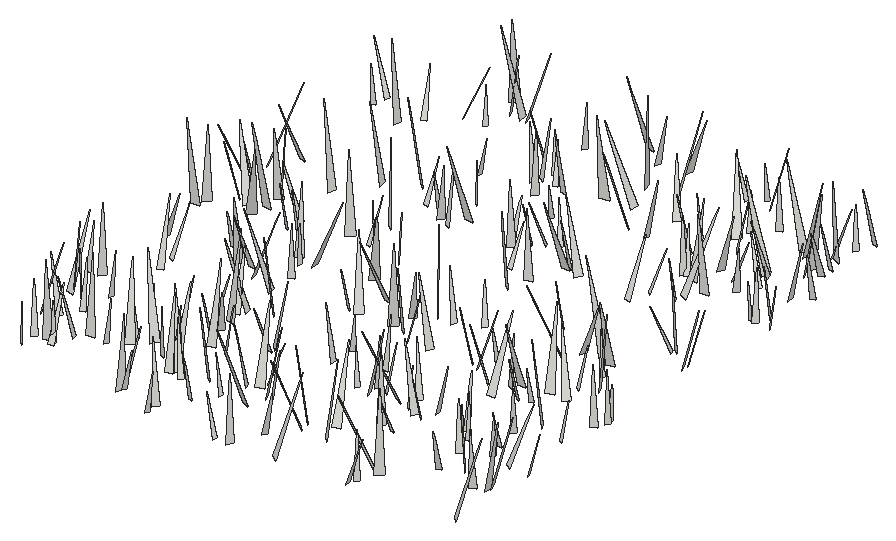
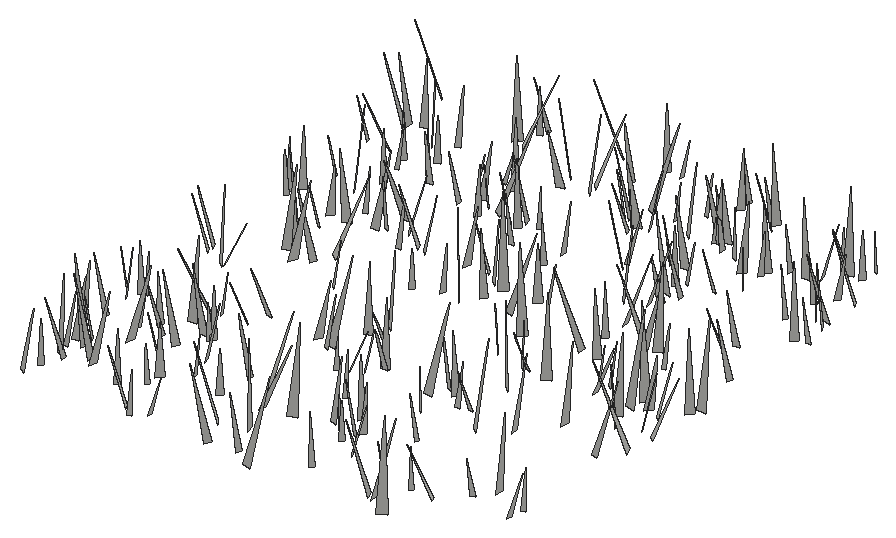
# SketchUp Ruby script. Lengths in inches.
U = 1.inch
M = Sketchup.active_model
def pt(a) = Geom::Point3d.new(a.map { |v| v * U })
def face(e, loops, mat)
  f = e.add_face(loops[0].map { |a| pt(a) })
  loops[1..].each { |l| e.add_face(l.map { |a| pt(a) }).erase! }
  f.material = f.back_material = mat if mat
  f
end
# faces: each face lists its corners as indices into pts; further lists are holes
def faces(e, pts, list, mat = nil) = list.each { |f| face(e, (f[0].is_a?(Array) ? f : [f]).map { |l| l.map { |i| pts[i] } }, mat) }
# xy, xz, yz: faces in a plane at the given z, y or x. An outline is a flat list of corners, or four numbers for a rectangle; further outlines are holes
def ring(l) = l.size == 4 ? [[l[0], l[1]], [l[2], l[1]], [l[2], l[3]], [l[0], l[3]]] : l.each_slice(2).to_a
def flat(e, list, mat, &to3) = list.each { |f| face(e, (f[0].is_a?(Array) ? f : [f]).map { |l| ring(l).map { |u, v| to3.(u, v) } }, mat) }
def xy(e, z, list, mat = nil) = flat(e, list, mat) { |x, y| [x, y, z] }
def xz(e, y, list, mat = nil) = flat(e, list, mat) { |x, z| [x, y, z] }
def yz(e, x, list, mat = nil) = flat(e, list, mat) { |y, z| [x, y, z] }
def lines(e, pts, list) = list.each { |a, b| e.add_line(pt(pts[a]), pt(pts[b])) }
# prism: a flat outline (further loops are holes) pulled along v
def prism(e, loops, v, mat = nil)
  f = face(e, loops, mat); d = Geom::Vector3d.new(v.map { |x| x * U })
  f.pushpull(f.normal.samedirection?(d) ? d.length : -d.length)
end
def box(e, o, s, mat = nil) = prism(e, [[o, [o[0] + s[0], o[1], o[2]], [o[0] + s[0], o[1] + s[1], o[2]], [o[0], o[1] + s[1], o[2]]]], [0, 0, s[2]], mat)
def at(x, y, z, deg = 0) = Geom::Transformation.translation(pt([x, y, z])) * Geom::Transformation.rotation(ORIGIN, Z_AXIS, deg.degrees)
def axes(o, x, y, z) = Geom::Transformation.new([*x, 0, *y, 0, *z, 0, *pt(o).to_a, 1])
def part(name) = M.definitions.add(name)
# library, detail: a bought-in or finely detailed component or shape, given as its bounding box
def library(name, o, s) = part(name).tap { |d| box(d.entities, o, s) }
def detail(e, o, s) = box(e.add_group.entities, o, s)
def put(e, d, t, mat = nil) = e.add_instance(d, t).tap { |i| i.material = mat if mat }
def group(e, t, mat = nil) = e.add_group.tap { |g| g.transformation = t; g.material = mat if mat }.entities
root = M.entities
c1 = part("fur_instance\#9")
p = [[0.8125,0,1.79],[0.67,-0.02,1.48],[0,-0.11,0],[0,0.11,0]]
faces(c1.entities,p,[[0,1,2,3]])
put(root,c1,axes([490.36,55.36,-21.66],[3.76138,-1.24538,0.93866],[-1.27843,-3.86595,-0.00634],[-0.89313,0.28885,3.96218]))
put(root,c1,axes([503.76,55.4,-21.66],[-3.79892,0.58903,0.61511],[0.5899,3.84804,-0.04166],[0.61427,-0.05255,3.84409]))
put(root,c1,axes([506.5,55.57,-21.66],[-5.0872,2.66073,2.45988],[2.85923,5.55214,-0.09239],[2.22604,-1.05084,5.74025]))
put(root,c1,axes([528.55,57.22,-21.66],[4.6292,0.17151,0.50537],[0.17521,-4.6565,-0.02456],[-0.5041,-0.0434,4.63231]))
put(root,c1,axes([482.875,58.1875,-21.66],[-5.61419,2.77509,3.47904],[3.15086,6.4338,-0.04739],[3.14276,-1.49299,6.26243]))
put(root,c1,axes([490.25,57.73,-21.66],[-4.38445,3.57185,1.79964],[3.76738,4.58485,0.07863],[1.34299,-1.20052,5.65467]))
put(root,c1,axes([514.83,56.21,-21.66],[4.48947,6.23838,0.89691],[6.27438,-4.52789,0.08708],[-0.59503,-0.67674,7.68539]))
put(root,c1,axes([483.18,58.77,-21.66],[3.78435,-1.32179,0.68035],[-1.35222,-3.83372,0.07338],[-0.61764,0.29457,4.00787]))
put(root,c1,axes([529.15,58.78,-21.66],[1.67153,-3.68103,1.97281],[-4.08391,-1.88531,-0.05752],[-0.87388,1.76964,4.04237]))
put(root,c1,axes([461.67,60.13,-21.66],[1.95949,2.80373,1.45551],[3.04239,-2.136,0.01872],[-0.85045,-1.18135,3.42055]))
put(root,c1,axes([548.44,58.8,-21.66],[5.3088,5.05785,1.00754],[5.10033,-5.36326,0.04959],[-0.76398,-0.65873,7.33231]))
put(root,c1,axes([482.64,59.66,-21.66],[3.62084,3.81527,1.03017],[3.87963,-3.69771,0.05854],[-0.75237,-0.70613,5.25959]))
put(root,c1,axes([508.8125,61.37,-21.66],[3.98619,-2.41358,0.43201],[-2.42835,-4.00018,0.05811],[-0.33929,0.27366,4.65958]))
put(root,c1,axes([528.84,63.33,-21.66],[-5.75391,-4.14909,0.07824],[-4.14913,5.75437,0.02082],[0.07564,0.02888,7.0938]))
put(root,c1,axes([493.09,62.62,-21.66],[-1.22069,-3.41408,1.05948],[-3.55821,1.26785,-0.01408],[0.34288,1.00256,3.62571]))
put(root,c1,axes([530.64,62.39,-21.66],[5.17413,-4.7343,3.23528],[-5.24163,-5.67192,0.08293],[-2.32507,2.25121,7.01272]))
put(root,c1,axes([464.33,63.53,-21.66],[2.05152,-6.96349,2.48946],[-7.36809,-2.14532,0.07104],[-0.63146,2.40909,7.25905]))
put(root,c1,axes([465.36,63.47,-21.66],[2.21811,-2.97156,1.30139],[-3.14682,-2.35396,-0.01147],[-0.78819,1.03561,3.7081]))
put(root,c1,axes([461.8,63.27,-21.66],[2.76185,-3.07557,2.49035],[-3.57907,-3.23702,-0.02845],[-1.68858,1.83068,4.13354]))
put(root,c1,axes([512.22,66.18,-21.66],[-4.64993,-4.92524,0.42817],[-4.93518,4.6591,-0.00251],[0.29211,0.31306,6.77347]))
put(root,c1,axes([465.56,62.57,-21.66],[-0.62554,4.99616,0.12365],[4.99768,0.62512,0.02455],[-0.009,-0.12574,5.03511]))
put(root,c1,axes([500.61,66.83,-21.66],[-3.23676,-6.95107,0.75182],[-6.9834,3.25434,0.02332],[0.33861,0.67166,7.66769]))
put(root,c1,axes([466.89,66.75,-21.66],[-4.90354,-1.85753,0.89414],[-1.8937,4.97041,-0.05944],[0.81474,0.37312,5.24324]))
put(root,c1,axes([517.3,66.01,-21.66],[-4.33935,-4.28478,3.74469],[-5.00881,5.11096,0.04388],[2.70071,2.59437,6.09815]))
put(root,c1,axes([496.04,66.59,-21.66],[-3.46887,0.5768,0.94943],[0.60796,3.5911,0.03958],[0.92978,-0.19616,3.51628]))
put(root,c1,axes([544.63,68.05,-21.66],[1.69924,-5.28596,1.58911],[-5.50046,-1.7602,0.02657],[-0.46001,1.5213,5.5523]))
put(root,c1,axes([511.7,68.27,-21.66],[-4.72321,-4.87597,2.05821],[-5.0831,4.94763,0.05633],[1.47426,1.43735,6.78828]))
put(root,c1,axes([536.71,69.47,-21.66],[2.00782,-4.43373,0.05819],[-4.43409,-2.00742,0.0429],[0.01508,0.0707,4.86698]))
put(root,c1,axes([487.84,66.88,-21.66],[-3.61656,3.24074,0.55892],[3.26072,3.64166,-0.01623],[0.42715,-0.36083,4.85609]))
put(root,c1,axes([471.99,68.38,-21.66],[-3.43259,1.11019,2.13702],[1.24058,4.00441,-0.08763],[2.06406,-0.56053,3.60659]))
put(root,c1,axes([485.18,67.19,-21.66],[-1.64071,6.20292,1.41522],[6.35653,1.66047,0.09149],[0.27128,-1.39198,6.41559]))
put(root,c1,axes([468.6,68.52,-21.66],[-0.16128,6.84934,2.86842],[7.42417,0.20732,-0.07764],[0.15166,-2.86546,6.8508]))
put(root,c1,axes([491.39,69.34,-21.66],[-4.35453,-4.53446,2.05004],[-4.74623,4.60317,0.10013],[1.49574,1.4055,6.28595]))
put(root,c1,axes([546.7,69.05,-21.66],[6.13024,0.22864,1.74835],[0.20896,-6.37456,0.10097],[-1.75081,0.03976,6.13367]))
put(root,c1,axes([484.33,69.59,-21.66],[5.43956,-0.0104,1.6458],[0.01524,-5.68242,-0.08629],[-1.64576,-0.087,5.43889]))
put(root,c1,axes([486.57,68.29,-21.66],[-5.17368,4.83178,0.63052],[4.85594,5.1888,0.08232],[0.40437,-0.49072,7.07858]))
put(root,c1,axes([485.625,68.45,-21.66],[0.08321,7.29137,1.2347],[7.39423,-0.10178,0.10277],[-0.11831,-1.23331,7.29112]))
put(root,c1,axes([481.32,70.5,-21.66],[-1.7362,-3.80786,1.79903],[-4.13168,1.91701,0.07019],[0.81577,1.60498,4.18441]))
put(root,c1,axes([546.71,70.23,-21.66],[6.30339,2.19635,1.13005],[2.22882,-6.39265,-0.00763],[-1.06457,-0.37914,6.67507]))
put(root,c1,axes([457.78,70.02,-21.66],[5.69643,3.12279,1.00252],[3.16084,-5.76326,-0.00802],[-0.87518,-0.48903,6.49623]))
put(root,c1,axes([497.28,71.32,-21.66],[-4.91949,-2.25789,1.34677],[-2.33985,5.06309,-0.05864],[1.19873,0.61667,5.41258]))
put(root,c1,axes([502.79,70.77,-21.66],[3.09566,2.75124,1.27433],[2.88928,-3.22895,-0.04754],[-0.91941,-0.88367,4.14127]))
put(root,c1,axes([501.86,70.49,-21.66],[5.547,2.87669,1.51326],[2.93945,-5.71712,0.09337],[-1.38744,-0.61131,6.24786]))
put(root,c1,axes([460.85,70.55,-21.66],[-4.64621,2.31988,0.55706],[2.32982,4.67441,-0.03457],[0.51391,-0.21773,5.19306]))
put(root,c1,axes([540.16,71.62,-21.66],[-4.40906,-3.22075,2.19411],[-3.50304,4.72714,-0.10035],[1.70765,1.38134,5.45921]))
put(root,c1,axes([474.79,70.5625,-21.66],[-3.82919,5.78151,1.38736],[5.88668,3.91838,-0.08139],[0.83523,-1.11076,6.93412]))
put(root,c1,axes([516.27,69.64,-21.66],[-1.83957,6.80237,0.25254],[6.80704,1.83779,0.08208],[-0.01336,-0.2652,7.04624]))
put(root,c1,axes([474.77,72.12,-21.66],[-3.91308,1.33626,1.31278],[1.41439,4.10109,0.04154],[1.2282,-0.46546,4.13474]))
put(root,c1,axes([523.81,74.12,-21.66],[-1.2303,-3.6424,0.32202],[-3.65502,1.23499,0.00478],[0.10759,0.30356,3.84457]))
put(root,c1,axes([499.16,72.21,-21.66],[-1.91608,6.79372,1.10059],[6.8739,1.94553,-0.04218],[0.33984,-1.04766,7.05863]))
put(root,c1,axes([477.66,73.1875,-21.66],[-6.04844,4.67756,1.28768],[4.75602,6.12308,0.0974],[0.95811,-0.86582,7.6455]))
put(root,c1,axes([499.44,74.11,-21.66],[4.10602,0.97464,0.35289],[0.9844,-4.11806,-0.08026],[-0.32469,-0.15985,4.21935]))
put(root,c1,axes([462.84,73.9,-21.66],[-1.62337,4.08317,1.17277],[4.21606,1.70273,-0.09236],[0.52201,-1.05424,4.39307]))
put(root,c1,axes([521.2,74.79,-21.66],[4.8811,-3.48072,2.77846],[-3.79933,-5.40519,-0.09683],[-2.32386,1.52607,5.99426]))
put(root,c1,axes([497.99,74.92,-21.66],[3.13012,3.09581,1.75638],[3.35561,-3.34662,-0.08138],[-1.18695,-1.29717,4.40172]))
put(root,c1,axes([535.99,75.43,-21.66],[-2.40866,3.6867,1.3913],[3.88066,2.50239,0.08743],[0.68406,-1.21467,4.40293]))
put(root,c1,axes([548.74,76.65,-21.66],[3.66327,1.41122,0.72087],[1.44956,-3.71776,-0.08822],[-0.64027,-0.34277,3.92471]))
put(root,c1,axes([474.44,76.95,-21.66],[2.40837,2.51325,1.53163],[2.71206,-2.66382,0.10655],[-1.14326,-1.0248,3.47927]))
put(root,c1,axes([459.59,77.56,-21.66],[3.22406,2.21993,1.84513],[2.48282,-3.54361,-0.0749],[-1.47248,-1.11442,3.91371]))
put(root,c1,axes([540.6,77.99,-21.66],[2.98723,-2.64764,1.00912],[-2.72025,-3.09017,-0.05514],[-0.79284,0.62671,3.99131]))
put(root,c1,axes([488.04,77.79,-21.66],[3.88099,1.49769,1.22771],[1.56049,-4.04689,0.00388],[-1.14683,-0.43823,4.15995]))
put(root,c1,axes([544.7,76.7,-21.66],[3.10305,4.72146,0.30771],[4.72969,-3.10544,-0.04628],[-0.13026,-0.28259,5.64969]))
put(root,c1,axes([485.26,77.65,-21.66],[-1.01475,7.09695,1.79918],[7.31311,1.06925,-0.09303],[0.3496,-1.76734,7.16853]))
put(root,c1,axes([457.64,77.19,-21.66],[1.8777,6.7714,0.98346],[6.8334,-1.90815,0.09124],[-0.35155,-0.923,7.02632]))
put(root,c1,axes([457.04,79.09,-21.66],[-4.37143,-2.8181,2.86453],[-3.24687,4.97094,-0.06453],[2.3675,1.61389,5.20067]))
put(root,c1,axes([518.65,82.21,-21.66],[-3.40543,-6.99905,0.02732],[-6.9991,3.40539,-0.01642],[-0.00281,0.03175,7.78353]))
put(root,c1,axes([534.7,79.28,-21.66],[-0.32853,3.96848,1.56907],[4.26678,0.33258,0.05223],[0.07349,-1.56822,3.98171]))
put(root,c1,axes([524.65,80.14,-21.66],[-2.53419,-2.69204,0.92744],[-2.77792,2.61003,-0.01451],[0.6248,0.68554,3.69715]))
put(root,c1,axes([539.68,80.83,-21.66],[0.38747,-3.62863,0.53891],[-3.66751,-0.39531,-0.02484],[-0.08219,0.53319,3.64917]))
put(root,c1,axes([463.42,80.24,-21.66],[4.19942,-1.36084,1.21546],[-1.38514,-4.36301,-0.09922],[-1.1877,0.2767,4.41329]))
put(root,c1,axes([493.17,82.1,-21.66],[-1.39577,-4.42794,0.41329],[-4.44248,1.40819,0.08395],[0.20461,0.36877,4.64196]))
put(root,c1,axes([481.99,81.34,-21.66],[-1.43466,-3.23484,0.82707],[-3.31328,1.49057,0.08262],[0.41278,0.72144,3.53774]))
put(root,c1,axes([523.16,80.42,-21.66],[-5.60882,2.54428,1.1021],[2.59069,5.69507,0.03704],[0.9881,-0.48955,6.15881]))
put(root,c1,axes([483.17,82.64,-21.66],[3.21105,-3.45107,0.18225],[-3.45172,-3.21492,-0.06213],[-0.16965,0.09106,4.71348]))
put(root,c1,axes([477.17,80.58,-21.66],[1.79566,3.71313,0.76849],[3.77743,-1.82574,-0.00496],[-0.33004,-0.69403,4.12452]))
put(root,c1,axes([513.52,81.33,-21.66],[5.7925,1.49056,1.34896],[1.52882,-5.93778,-0.00376],[-1.30544,-0.3399,5.9812]))
put(root,c1,axes([510.75,81.73,-21.66],[-2.66914,2.15187,1.53787],[2.38339,2.90414,0.07299],[1.14676,-1.02728,3.42776]))
put(root,c1,axes([521.08,81.5,-21.66],[-2.34168,-2.41248,1.9117],[-2.76899,2.70012,0.01564],[1.3444,1.35921,3.36204]))
put(root,c1,axes([532.76,81.25,-21.66],[-0.41482,4.98169,1.32883],[5.15587,0.40286,0.09923],[0.00793,-1.33251,4.99795]))
put(root,c1,axes([513.65,83.53,-21.66],[4.04014,-3.74392,1.13553],[-3.80741,-4.13804,-0.09691],[-0.90002,0.69913,5.50729]))
put(root,c1,axes([525.59,83.125,-21.66],[4.33952,0.70183,1.00017],[0.70812,-4.45199,0.05164],[-0.99573,-0.10739,4.3956]))
put(root,c1,axes([515.52,83,-21.66],[2.94995,3.39967,1.09614],[3.50655,-3.02709,-0.04841],[-0.68072,-0.86052,4.50085]))
put(root,c1,axes([493.18,83.31,-21.66],[-3.61899,-3.55384,3.43713],[-4.24844,4.41399,0.09065],[2.52873,2.32973,5.07136]))
put(root,c1,axes([458.0625,84.67,-21.66],[-4.38219,4.14776,3.28171],[4.71988,4.98997,-0.0042],[2.38668,-2.25242,6.03386]))
put(root,c1,axes([455.79,84.19,-21.66],[0.08928,4.21713,1.27448],[4.4055,-0.088,-0.01741],[-0.00879,-1.27457,4.21804]))
put(root,c1,axes([538.54,85.59,-21.66],[2.93376,-3.22318,1.07266],[-3.3076,-3.03341,-0.06853],[-0.77414,0.74566,4.35788]))
put(root,c1,axes([480.125,85.17,-21.66],[4.64255,0.07182,0.51653],[0.0806,-4.67045,-0.07504],[-0.51523,-0.08349,4.6425]))
put(root,c1,axes([520.78,84.6,-21.66],[-3.74669,3.50171,1.17991],[3.59906,3.83892,0.03541],[0.8372,-0.8322,5.12819]))
put(root,c1,axes([502.92,85.64,-21.66],[-4.88413,-0.13594,1.40409],[-0.16648,5.08029,-0.08723],[1.4008,0.12978,4.88524]))
put(root,c1,axes([482.7,85.53,-21.66],[2.51079,7.35519,2.45383],[7.71335,-2.63218,-0.00261],[-0.79014,-2.32314,7.77193]))
put(root,c1,axes([546.01,87.9,-21.66],[1.71748,3.11444,0.84575],[3.20742,-1.75327,-0.057],[-0.35706,-0.7688,3.55615]))
put(root,c1,axes([511.01,88.48,-21.66],[0.37459,4.6587,1.44665],[4.87681,-0.39143,-0.00226],[-0.11359,-1.44218,4.67373]))
put(root,c1,axes([482.69,89.75,-21.66],[-6.22564,-1.43503,0.72375],[-1.44178,6.26598,0.02194],[0.71021,0.14105,6.38885]))
put(root,c1,axes([540.74,90.06,-21.66],[-6.29622,-3.82649,2.40942],[-4.00808,6.63484,0.06324],[2.09347,1.19444,7.36752]))
put(root,c1,axes([503.11,90.23,-21.66],[2.68413,-2.59886,0.79499],[-2.66781,-2.73276,0.07385],[-0.51851,0.60713,3.7354]))
put(root,c1,axes([481.82,88,-21.66],[-1.75814,5.2069,0.13379],[5.20853,1.75836,0.01288],[0.0306,-0.13088,5.4957]))
put(root,c1,axes([486.38,91.625,-21.66],[-4.69837,-4.55111,2.1601],[-4.81656,4.92378,-0.10244],[1.47629,1.58022,6.5404]))
put(root,c1,axes([463.86,91.76,-21.66],[-1.14776,6.0133,0.84328],[6.0716,1.14805,0.07727],[0.08148,-0.84289,6.12137]))
put(root,c1,axes([532.56,94.19,-21.66],[-2.07432,-2.92088,0.84042],[-3.01146,2.11274,-0.09003],[0.41107,0.73854,3.58137]))
put(root,c1,axes([534.76,94.75,-21.66],[1.50784,-3.41822,0.5063],[-3.4457,-1.52893,-0.06057],[-0.26023,0.4385,3.73552]))
put(root,c1,axes([525.6,95.48,-21.66],[-4.16981,-3.31895,0.85743],[-3.36405,4.22145,-0.01946],[0.65859,0.54939,5.32938]))
put(root,c1,axes([547.18,94.74,-21.66],[2.70237,-4.42657,2.31196],[-4.83243,-2.98105,-0.05917],[-1.25989,1.93941,5.18593]))
put(root,c1,axes([528.59,92.39,-21.66],[0.11708,7.08162,0.20269],[7.08451,-0.11681,-0.01106],[0.00771,-0.20285,7.08258]))
put(root,c1,axes([530.49,97.76,-21.66],[-0.18064,-6.52008,0.8881],[-6.57997,0.17015,-0.08916],[-0.06535,0.89016,6.52198]))
put(root,c1,axes([481.57,96.98,-21.66],[-7.05109,-1.52018,0.70264],[-1.52291,7.08527,0.04653],[0.69669,0.10238,7.21295]))
put(root,c1,axes([548.23,96.78,-21.66],[-3.98978,2.11987,2.03955],[2.3526,4.36264,0.06771],[1.76604,-1.02247,4.51748]))
put(root,c1,axes([463.33,95.2,-21.66],[1.79121,4.66243,0.42191],[4.67903,-1.79759,0.00003],[-0.15134,-0.39383,4.99466]))
put(root,c1,axes([529.24,96.56,-21.66],[1.95895,3.98258,1.69888],[4.26762,-2.09086,-0.01944],[-0.73116,-1.53362,4.43825]))
put(root,c1,axes([548,97.8,-21.66],[2.54214,-2.62214,0.84113],[-2.70032,-2.59808,0.06187],[-0.53981,0.64801,3.65161]))
put(root,c1,axes([519.99,98.7,-21.66],[-3.55733,-3.55392,1.20149],[-3.66341,3.64755,-0.05732],[0.80828,0.89081,5.02808]))
put(root,c1,axes([508.05,97.625,-21.66],[3.92442,2.27765,0.90763],[2.32456,-4.0011,-0.01041],[-0.77966,-0.46478,4.53747]))
put(root,c1,axes([512.18,97.91,-21.66],[-5.92125,2.00992,1.02968],[2.02644,6.00419,-0.06686],[0.99676,-0.26678,6.25272]))
put(root,c1,axes([521.57,97.98,-21.66],[5.13146,2.31605,0.71954],[2.33013,-5.17519,0.0403],[-0.67253,-0.25897,5.62978]))
put(root,c1,axes([472.16,100.7,-21.66],[3.11086,-6.46121,1.0779],[-6.53922,-3.13316,0.09147],[-0.38422,1.01124,7.17051]))
put(root,c1,axes([474.56,101.08,-21.66],[-0.49515,-5.81147,0.35136],[-5.82208,0.49376,-0.03799],[-0.0081,0.35331,5.8324]))
put(root,c1,axes([503,100.38,-21.66],[4.71718,-6.41333,2.08506],[-6.64537,-4.85367,0.10513],[-1.14777,1.74389,7.96063]))
put(root,c1,axes([505.4,99.68,-21.66],[-3.42106,-4.15596,2.05732],[-4.44833,3.66341,0.00339],[1.31032,1.58608,5.3829]))
put(root,c1,axes([523.79,100.25,-21.66],[0.76269,-3.95415,0.89534],[-4.04548,-0.80213,-0.09639],[-0.26648,0.86018,4.02588]))
put(root,c1,axes([476.5625,98.93,-21.66],[6.39935,1.66924,0.57136],[1.67346,-6.42366,0.02366],[-0.55885,-0.12123,6.61343]))
put(root,c1,axes([494.44,100.16,-21.66],[-1.9321,-3.03286,0.9193],[-3.13143,1.99261,-0.00754],[0.48737,0.77951,3.596]))
put(root,c1,axes([538.63,98.55,-21.66],[-4.40287,4.25609,0.42122],[4.26988,4.40886,0.08361],[0.24458,-0.35298,6.12311]))
put(root,c1,axes([457.97,100.76,-21.66],[4.67852,-1.7119,0.20248],[-1.71617,-4.68064,0.08066],[-0.16239,0.14538,4.98123]))
put(root,c1,axes([535.25,98.8,-21.66],[-2.63415,6.93544,1.64719],[7.09873,2.71215,-0.06728],[0.64926,-1.51533,7.41852]))
put(root,c1,axes([496.4375,100.07,-21.66],[-4.20959,5.12778,0.85898],[5.1677,4.24809,-0.03415],[0.57165,-0.64206,6.63427]))
put(root,c1,axes([481.34,102.2,-21.66],[2.46407,-3.91283,1.91735],[-4.25122,-2.64198,0.07181],[-0.95581,1.66367,4.6235]))
put(root,c1,axes([503.83,104.2,-21.66],[4.00821,-3.73033,0.31245],[-3.73197,-4.01777,-0.09299],[-0.29215,0.14465,5.47471]))
put(root,c1,axes([497.75,105.61,-21.66],[-1.99035,-6.59495,0.1128],[-6.59501,1.99173,0.07994],[0.10913,0.08488,6.88828]))
put(root,c1,axes([537.77,102.44,-21.66],[1.92341,3.31368,0.82854],[3.39872,-1.95136,-0.08567],[-0.34002,-0.7604,3.83049]))
put(root,c1,axes([468.19,104.3,-21.66],[0.55845,-3.67703,0.59896],[-3.72525,-0.55803,0.04757],[-0.0423,0.59936,3.71889]))
put(root,c1,axes([540.7,104.22,-21.66],[5.91365,2.78735,2.33328],[2.94924,-6.28377,0.03183],[-2.12497,-0.96423,6.53755]))
put(root,c1,axes([530,108.43,-21.66],[-4.57477,-6.03245,0.25242],[-6.03633,4.57654,-0.02819],[0.13005,0.21817,7.57088]))
put(root,c1,axes([479.83,106.31,-21.66],[-3.27969,0.65416,1.38528],[0.68941,3.5533,-0.04576],[1.36808,-0.22237,3.34398]))
put(root,c1,axes([506.58,107.02,-21.66],[-5.8561,-4.67693,3.47291],[-5.12361,6.47844,0.0849],[2.77191,2.09401,7.49403]))
put(root,c1,axes([509.93,106.72,-21.66],[-4.33048,1.8912,1.2808],[1.94847,4.49129,-0.04381],[1.19187,-0.47097,4.72523]))
put(root,c1,axes([481.6875,107.62,-21.66],[7.09843,0.26187,0.16049],[0.26265,-7.10014,-0.03187],[-0.15921,-0.03777,7.10319]))
put(root,c1,axes([538.4,107.76,-21.66],[-3.29969,1.99263,1.18367],[2.06312,3.46364,-0.07948],[1.05601,-0.54058,3.85386]))
put(root,c1,axes([491.65,109.82,-21.66],[5.04429,-5.44094,0.7168],[-5.46997,-5.06343,0.05905],[-0.44381,0.56596,7.41924]))
put(root,c1,axes([478.23,108.16,-21.66],[-2.28357,5.70644,2.33564],[6.0895,2.47813,-0.10083],[0.96778,-2.12809,6.14557]))
put(root,c1,axes([514.42,108.79,-21.66],[-2.6188,2.85202,1.01974],[2.95253,2.70449,0.01846],[0.67563,-0.76402,3.87193]))
put(root,c1,axes([537.0625,111.28,-21.66],[1.68994,-6.65431,0.98946],[-6.7239,-1.70391,0.02495],[-0.21912,0.96522,6.8655]))
put(root,c1,axes([455.31,111.17,-21.66],[-0.06707,-7.91469,2.47451],[-8.29222,0.04381,-0.08466],[-0.06773,2.47503,7.91452]))
put(root,c1,axes([531.44,111.65,-21.66],[5.62437,-1.82953,0.08499],[-1.8284,-5.62476,-0.0835],[-0.10665,-0.05312,5.91386]))
put(root,c1,axes([463.97,114.14,-21.66],[5.44226,-5.9088,0.26751],[-5.91243,-5.44486,0.01623],[-0.16928,0.20777,8.03317]))
put(root,c1,axes([456.17,112.94,-21.66],[-4.86484,4.13925,3.64162],[4.78109,5.5858,0.03796],[2.74517,-2.39309,6.38738]))
put(root,c1,axes([471.11,113.91,-21.66],[-2.39364,-3.13142,1.17859],[-3.27618,2.48779,-0.04385],[0.67935,0.9641,3.94124]))
put(root,c1,axes([534.29,113.26,-21.66],[-8.05212,1.79962,1.36323],[1.82873,8.16018,0.02927],[1.32393,-0.32629,8.25072]))
put(root,c1,axes([473.27,114.06,-21.66],[-3.37227,-0.8607,0.92289],[-0.91034,3.4828,-0.07828],[0.87397,0.30665,3.4795]))
put(root,c1,axes([464.56,117.11,-21.66],[-1.19832,-8.06423,2.00487],[-8.30399,1.23724,0.01324],[0.30817,1.98109,8.15276]))
put(root,c1,axes([524,116.06,-21.66],[-2.56443,-3.19615,1.19823],[-3.34404,2.653,-0.08027],[0.6845,0.98675,4.09698]))
put(root,c1,axes([459.35,116.92,-21.66],[-3.89073,-3.2521,0.98713],[-3.3181,3.95947,-0.03367],[0.73538,0.65937,5.07078]))
put(root,c1,axes([491.41,116.3,-21.66],[3.14318,2.78213,1.66083],[2.96777,-3.40061,0.07991],[-1.30037,-1.03624,4.19683]))
put(root,c1,axes([471.76,116.71,-21.66],[-5.15429,0.32159,0.0951],[0.32057,5.15491,-0.05731],[0.09848,0.05128,5.164]))
put(root,c1,axes([461.82,115.89,-21.66],[-5.31881,4.24046,0.31909],[4.24772,5.322,0.07866],[0.20039,-0.26047,6.80184]))
put(root,c1,axes([485.46,117.6875,-21.66],[-2.49049,-3.07283,1.62396],[-3.33154,2.67981,-0.03854],[0.99012,1.28779,3.95516]))
put(root,c1,axes([480.12,118.32,-21.66],[4.03772,-5.94106,3.0996],[-6.44975,-4.42725,-0.08397],[-1.8178,2.512,7.18278]))
put(root,c1,axes([546.38,117.58,-21.66],[4.95919,2.18923,1.00137],[2.21006,-5.04934,0.09393],[-0.95452,-0.31696,5.4201]))
put(root,c1,axes([484.25,117.62,-21.66],[1.13394,4.06883,0.24777],[4.07369,-1.14042,0.08414],[-0.14769,-0.216,4.22305]))
put(root,c1,axes([464.42,120.27,-21.66],[2.81734,-6.20209,1.85033],[-6.41792,-2.93797,-0.07572],[-0.83667,1.65211,6.81158]))
put(root,c1,axes([546.32,119.05,-21.66],[4.35259,2.65064,0.87547],[2.69973,-4.40951,-0.0717],[-0.70982,-0.51745,5.09567]))
put(root,c1,axes([541.75,120.71,-21.66],[-3.79405,-1.81524,0.00607],[-1.81515,3.79397,0.03081],[0.01877,-0.02517,4.20582]))
put(root,c1,axes([509.16,120.71,-21.66],[3.99412,4.65299,3.2629],[5.30006,-4.48907,-0.08624],[-2.05092,-2.53923,6.13155]))
put(root,c1,axes([458.83,121.31,-21.66],[-4.42725,-2.60663,1.07476],[-2.66002,4.52485,0.01676],[0.93485,0.53053,5.13759]))
put(root,c1,axes([455.86,122.57,-21.66],[-3.26059,-4.43586,0.10579],[-4.43536,3.26207,0.0775],[0.12511,0.03932,5.50476]))
put(root,c1,axes([542.23,121.18,-21.66],[-4.17203,-5.0841,2.64194],[-5.48144,4.49304,-0.00972],[1.66784,2.04897,6.57676]))
put(root,c1,axes([462.82,123.03,-21.66],[4.34542,2.75412,2.00138],[2.98226,-4.64462,-0.0836],[-1.6422,-1.14703,5.14401]))
put(root,c1,axes([510.52,124.35,-21.66],[-1.61639,5.70202,2.80279],[6.31476,1.76115,0.05886],[0.70173,-2.71416,5.92641]))
put(root,c1,axes([483.26,124.19,-21.66],[4.5767,5.68819,3.18986],[6.17982,-5.02762,0.09872],[-2.08339,-2.41752,7.30013]))
put(root,c1,axes([505.85,125.57,-21.66],[0.74131,3.87524,0.12897],[3.87698,-0.74271,0.03187],[-0.05555,-0.12068,3.94537]))
put(root,c1,axes([469.18,127.46,-21.66],[-7.46216,1.5868,2.36089],[1.65538,7.81249,-0.01867],[2.31332,-0.47194,7.62898]))
put(root,c1,axes([512.72,130.91,-21.66],[-0.43608,-7.58063,0.50958],[-7.59761,0.43802,0.01424],[0.04352,0.50791,7.59315]))
put(root,c1,axes([456.28,128.02,-21.66],[7.55875,3.30018,0.58934],[3.3113,-7.57673,-0.04195],[-0.52327,-0.27436,8.24768]))
put(root,c1,axes([459.4,132.41,-21.66],[-1.29873,-6.18935,0.13887],[-6.18983,1.30082,0.08883],[0.11547,0.11765,6.32352]))
put(root,c1,axes([487.88,131.01,-21.66],[4.42383,-2.92058,1.2942],[-2.99041,-4.56361,-0.07677],[-1.12348,0.64702,5.30039]))
put(root,c1,axes([490.07,129.9,-21.66],[-1.46329,-3.87448,2.4887],[-4.52721,1.6881,-0.03379],[0.84239,2.34204,4.14146]))
put(root,c1,axes([501.87,131.01,-21.66],[2.29625,-5.32789,2.30917],[-5.72704,-2.48806,-0.04565],[-0.95905,2.10109,5.80148]))
put(root,c1,axes([513.0625,131.5625,-21.66],[-1.72033,-4.15588,1.09836],[-4.2769,1.77348,0.01157],[0.4311,1.01028,4.49785]))
put(root,c1,axes([515.79,130.09,-21.66],[-6.07575,2.79462,0.62219],[2.80321,6.10345,-0.04049],[0.58225,-0.22305,6.68752]))
put(root,c1,axes([491.56,133.3,-21.66],[-1.16201,-7.65185,1.0654],[-7.72512,1.16361,-0.06847],[0.09162,1.06366,7.73928]))
put(root,c1,axes([526.125,129.2,-21.66],[0.97806,5.36378,0.25201],[5.36787,-0.98334,0.09641],[-0.14015,-0.23057,5.45137]))
put(root,c1,axes([501.68,131.18,-21.66],[0.3484,4.1984,0.59349],[4.23915,-0.35779,0.04247],[-0.09183,-0.58788,4.21262]))
put(root,c1,axes([485.5,133.69,-21.66],[0.8315,-3.67241,0.7269],[-3.73531,-0.86356,-0.09004],[-0.24991,0.6885,3.76429]))
put(root,c1,axes([503.7,133.61,-21.66],[2.36967,1.89121,2.13493],[2.35412,-2.86396,-0.07595],[-1.61018,-1.40392,3.03088]))
put(root,c1,axes([532.14,133.46,-21.66],[-3.28529,-1.60429,1.12724],[-1.66632,3.44368,0.04462],[1.03333,0.45264,3.6558]))
put(root,c1,axes([473.92,134,-21.66],[-6.8866,-1.44069,2.04712],[-1.4724,7.17733,0.09795],[2.02444,0.3193,7.035]))
put(root,c1,axes([505.68,134.73,-21.66],[-3.47734,-1.80435,0.22841],[-1.8088,3.48242,-0.02761],[0.19,0.12974,3.9175]))
put(root,c1,axes([527.41,133.07,-21.66],[2.54826,3.20038,0.28055],[3.20908,-2.5526,-0.02947],[-0.15164,-0.23787,4.09087]))
put(root,c1,axes([483.3,133.12,-21.66],[0.89706,4.01856,0.51185],[4.05094,-0.89322,-0.08685],[-0.02607,-0.51851,4.11655]))
put(root,c1,axes([545.09,135.93,-21.66],[-0.48209,-3.49328,1.24378],[-3.69826,0.54426,0.09516],[0.26993,1.21786,3.5251]))
put(root,c1,axes([546.02,136.08,-21.66],[-2.69115,3.5868,1.84623],[3.86426,2.92918,-0.05799],[1.15809,-1.43902,4.48375]))
put(root,c1,axes([548.86,136.08,-21.66],[-2.22453,-2.28888,1.93607],[-2.6411,2.63697,0.08289],[1.41842,1.32035,3.19071]))
put(root,c1,axes([479,137.47,-21.66],[-5.20637,-5.83633,2.28098],[-6.06397,5.44004,0.07832],[1.57922,1.64775,7.82067]))
put(root,c1,axes([507.56,135.95,-21.66],[-2.46678,3.0111,0.36551],[3.02886,2.4705,0.08915],[0.1623,-0.33942,3.8915]))
put(root,c1,axes([534.27,138.14,-21.66],[0.04247,-7.07988,2.41623],[-7.48051,-0.06275,-0.05238],[-0.06984,2.41579,7.07981]))
put(root,c1,axes([489.21,138.11,-21.66],[-2.0645,-2.99831,1.70133],[-3.28642,2.31061,0.08412],[1.04107,1.34824,3.63936]))
put(root,c1,axes([547.11,138.47,-21.66],[-3.81411,-2.18756,1.38745],[-2.30966,3.98998,-0.05835],[1.17299,0.74331,4.39652]))
put(root,c1,axes([532.3125,135.35,-21.66],[2.76635,7.35948,0.05567],[7.35952,-2.76581,-0.07342],[0.04914,-0.07794,7.86188]))
put(root,c1,axes([500.875,142.03,-21.66],[2.15592,-3.18911,0.31319],[-3.19535,-2.16794,-0.07942],[-0.24138,0.21478,3.84865]))
put(root,c1,axes([528.03,140.68,-21.66],[-3.99726,2.72851,1.81883],[2.89094,4.28575,-0.07581],[1.5477,-0.9584,4.83912]))
put(root,c1,axes([537.71,141.71,-21.66],[-2.80028,2.24736,2.49663],[2.73085,3.4158,-0.01176],[1.95607,-1.55147,3.59055]))
put(root,c1,axes([530.31,140.22,-21.66],[0.3651,6.79595,1.75212],[7.01816,-0.34958,-0.10649],[0.01583,-1.75528,6.80491]))
put(root,c1,axes([528.58,140.93,-21.66],[-2.41477,3.3901,0.55663],[3.41153,2.44646,-0.10002],[0.40504,-0.3947,4.161]))
put(root,c1,axes([535.15,144.35,-21.66],[4.26673,-0.51352,0.23406],[-0.5171,-4.27238,0.05285],[-0.22604,0.08052,4.29719]))
put(root,c1,axes([531.66,145.45,-21.66],[5.79925,-1.98106,0.58125],[-1.98372,-5.82701,-0.06806],[-0.57211,0.1232,6.12791]))
put(root,c1,axes([545.76,144.96,-21.66],[5.31059,0.52385,1.16283],[0.52648,-5.43598,0.04446],[-1.16164,-0.06886,5.33618]))
put(root,c1,axes([483.73,145.85,-21.66],[3.66443,-1.25509,0.51627],[-1.25966,-3.69872,-0.05095],[-0.50503,0.11865,3.87307]))
put(root,c1,axes([539.72,144.69,-21.66],[-3.84574,2.31871,0.01808],[2.31862,3.84577,-0.02193],[0.02681,0.00945,4.49062]))
put(root,c1,axes([494.51,145.94,-21.66],[4.30224,-3.16543,2.15858],[-3.43037,-4.62804,0.05027],[-1.70646,1.32286,5.34104]))
put(root,c1,axes([511.87,147.25,-21.66],[-4.79453,-5.10071,1.01007],[-5.15614,4.84133,-0.02673],[0.67211,0.75447,7.00029]))
put(root,c1,axes([524.97,146.3,-21.66],[-4.98874,-1.77944,1.14235],[-1.81158,5.1064,0.04294],[1.09068,0.3424,5.29642]))
put(root,c1,axes([548.35,147.23,-21.66],[1.07632,-4.38935,0.89904],[-4.4763,-1.09335,0.02097],[-0.19334,0.87825,4.51934]))
put(root,c1,axes([516.25,146.36,-21.66],[5.41159,0.09186,1.28906],[0.07062,-5.56242,0.09991],[-1.29039,0.08081,5.41145]))
put(root,c1,axes([538.75,148.3,-21.66],[-4.66141,-1.64687,0.68606],[-1.65466,4.70851,0.06011],[0.66704,0.1713,4.94341]))
put(root,c1,axes([497.46,149.29,-21.66],[-1.75963,-5.21212,1.71135],[-5.46295,1.82898,-0.04671],[0.50104,1.63703,5.50093]))
put(root,c1,axes([537.97,148.76,-21.66],[-8.02945,1.44749,0.94959],[1.4539,8.08421,-0.0293],[0.93976,-0.13944,8.15883]))
put(root,c1,axes([491.58,149.19,-21.66],[-4.02288,2.74208,1.38872],[2.85785,4.17888,0.02734],[1.13147,-0.80565,4.86845]))
put(root,c1,axes([463.69,150.51,-21.66],[-6.94561,0.7265,2.56424],[0.79665,7.39636,0.06233],[2.54332,-0.33278,6.98322]))
put(root,c1,axes([503.6,151.74,-21.66],[1.30407,-7.61557,2.3618],[-7.95747,-1.39423,-0.10194],[-0.50366,2.30972,7.72574]))
put(root,c1,axes([495.13,150.28,-21.66],[-1.61358,3.38665,0.61033],[3.4322,1.63258,0.01498],[0.24881,-0.55751,3.75138]))
put(root,c1,axes([523.21,151.14,-21.66],[-3.75742,-0.36081,1.22113],[-0.40687,3.94545,-0.08619],[1.20657,0.20686,3.77372]))
put(root,c1,axes([492.12,150.49,-21.66],[2.52877,4.50107,1.40807],[4.66336,-2.62485,0.01569],[-0.70386,-1.21962,5.16276]))
put(root,c1,axes([544.91,153.75,-21.66],[1.17594,-4.92519,0.34785],[-4.93492,-1.18388,-0.07952],[-0.1583,0.31979,5.06301]))
put(root,c1,axes([542.87,152.01,-21.66],[3.30994,1.56111,0.94089],[1.62723,-3.40964,-0.0672],[-0.82125,-0.46405,3.659]))
put(root,c1,axes([529.89,151.65,-21.66],[3.54809,3.00738,1.07129],[3.07779,-3.64774,0.04651],[-0.84804,-0.65624,4.65093]))
put(root,c1,axes([457.1,152.78,-21.66],[1.04159,-3.44564,1.2731],[-3.64709,-1.12789,-0.06873],[-0.4381,1.19732,3.59897]))
put(root,c1,axes([508.86,152.55,-21.66],[-7.40149,0.22253,0.007],[0.22253,7.40149,0.00759],[0.00677,-0.0078,7.40483]))
put(root,c1,axes([492.89,152.94,-21.66],[1.88047,-2.78184,1.95652],[-3.20631,-2.19563,-0.04014],[-1.13412,1.59479,3.35756]))
put(root,c1,axes([542.47,154.27,-21.66],[7.05562,-2.47543,1.6862],[-2.53392,-7.23407,-0.01726],[-1.59697,0.54154,7.47725]))
put(root,c1,axes([516.67,153.36,-21.66],[-3.66348,3.88372,0.60062],[3.90017,3.69385,-0.09601],[0.48235,-0.37054,5.33808]))
put(root,c1,axes([488.92,155.5,-21.66],[-3.66395,-2.75565,0.79106],[-2.79858,3.7164,-0.01609],[0.62239,0.48852,4.58453]))
put(root,c1,axes([544.86,156.09,-21.66],[-0.84306,-4.44176,0.86686],[-4.52258,0.85891,0.00263],[0.16427,0.85115,4.52106]))
put(root,c1,axes([466.31,153.88,-21.66],[-1.50833,4.20798,0.27956],[4.21722,1.50618,0.08227],[0.01672,-0.29093,4.46939]))
put(root,c1,axes([457.63,155.61,-21.66],[-4.98087,1.16288,0.32288],[1.15979,4.99131,-0.08543],[0.33384,0.00996,5.1141]))
put(root,c1,axes([527.28,154.77,-21.66],[-4.42637,5.44798,0.10976],[5.44745,4.42761,-0.08267],[0.13338,-0.03304,7.019]))
put(root,c1,axes([539.19,156.96,-21.66],[7.16515,0.1083,1.44204],[0.09788,-7.3087,0.06254],[-1.44279,0.042,7.1657]))
put(root,c1,axes([527.66,157.58,-21.66],[1.56835,-2.82264,1.69633],[-3.20586,-1.73838,0.07137],[-0.75322,1.52161,3.2283]))
put(root,c1,axes([474.875,158.3,-21.66],[-2.3678,2.48019,1.72309],[2.76192,2.66404,-0.03926],[1.22155,-1.2159,3.42875]))
put(root,c1,axes([537.98,158.04,-21.66],[-7.39383,1.79038,1.19471],[1.82356,7.48136,0.07416],[1.14343,-0.35412,7.60715]))
put(root,c1,axes([543.77,158.8125,-21.66],[2.87262,5.81566,3.24646],[6.49078,-3.23727,0.05584],[-1.49368,-2.88298,6.48619]))
put(root,c1,axes([506.33,158.89,-21.66],[7.01213,2.59998,3.36264],[2.81322,-7.70163,0.08845],[-3.18638,-1.07803,7.47811]))
put(root,c1,axes([470.45,158.51,-21.66],[4.47916,2.33614,0.04477],[2.33654,-4.47877,-0.05982],[-0.01203,-0.07375,5.05142]))
put(root,c1,axes([542.66,159.4,-21.66],[5.19271,0.37939,0.34653],[0.38191,-5.20401,-0.02543],[-0.34375,-0.05067,5.20649]))
put(root,c1,axes([530.99,160.69,-21.66],[1.68942,-4.24341,1.91691],[-4.60334,-1.82876,0.00876],[-0.70022,1.78447,4.56734]))
put(root,c1,axes([511.6,160.13,-21.66],[5.53821,4.98185,1.27941],[5.04776,-5.62536,0.05401],[-0.98782,-0.81487,7.449]))
put(root,c1,axes([491.43,162.16,-21.66],[3.58428,-2.61771,1.24135],[-2.70899,-3.7283,-0.04015],[-1.02701,0.69843,4.43823]))
put(root,c1,axes([544.11,163.15,-21.66],[-2.72992,2.63061,1.69887],[2.87463,2.99911,-0.02472],[1.24209,-1.1593,3.79104]))
put(root,c1,axes([477.83,163.92,-21.66],[-7.83982,-0.95667,1.33619],[-0.96404,7.9519,0.03699],[1.33088,0.12461,7.89789]))
put(root,c1,axes([475.53,163.7,-21.66],[4.582,2.26461,1.64468],[2.3704,-4.81752,0.02956],[-1.48816,-0.70087,5.111]))
put(root,c1,axes([478.9,163.63,-21.66],[6.34041,1.92452,0.88463],[1.94009,-6.39712,0.01179],[-0.84995,-0.24555,6.62604]))
put(root,c1,axes([521.17,165.05,-21.66],[-3.91396,0.19988,0.40503],[0.19284,3.93443,-0.07818],[0.40843,0.05784,3.91828]))
put(root,c1,axes([503.17,165.48,-21.66],[4.73571,-1.08461,0.9225],[-1.0987,-4.82145,-0.02851],[-0.90568,0.17765,4.85824]))
put(root,c1,axes([508.71,166.25,-21.66],[6.16535,-1.94029,0.16764],[-1.94054,-6.16752,-0.01601],[-0.16472,0.03505,6.46343]))
put(root,c1,axes([545.17,166.49,-21.66],[-1.95958,-4.83915,1.26512],[-4.97855,2.01787,0.00704],[0.48156,1.1699,5.22085]))
put(root,c1,axes([473.6875,167.09,-21.66],[3.80262,-6.94068,2.14426],[-7.19034,-3.9408,-0.00453],[-1.0344,1.87826,7.9141]))
put(root,c1,axes([525.47,165.35,-21.66],[4.69542,3.0157,0.91715],[3.05189,-4.76105,0.03053],[-0.78841,-0.46959,5.58037]))
put(root,c1,axes([499.41,168.36,-21.66],[-2.16653,-7.31637,0.90738],[-7.36569,2.18851,0.05952],[0.3151,0.85299,7.63018]))
put(root,c1,axes([523.5,167.05,-21.66],[1.81522,-3.21568,0.8696],[-3.29805,-1.87418,-0.04607],[-0.46866,0.73395,3.69235]))
